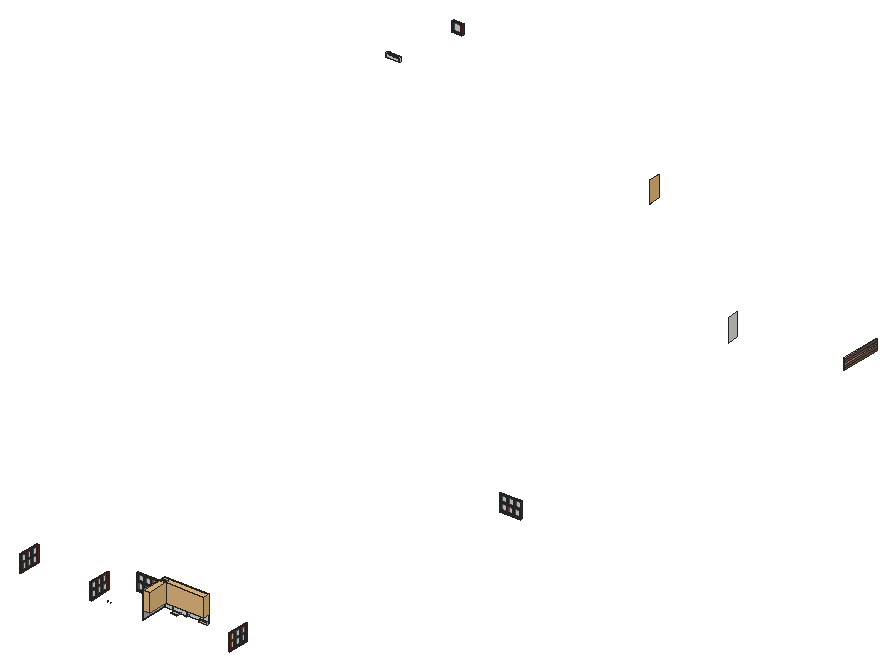
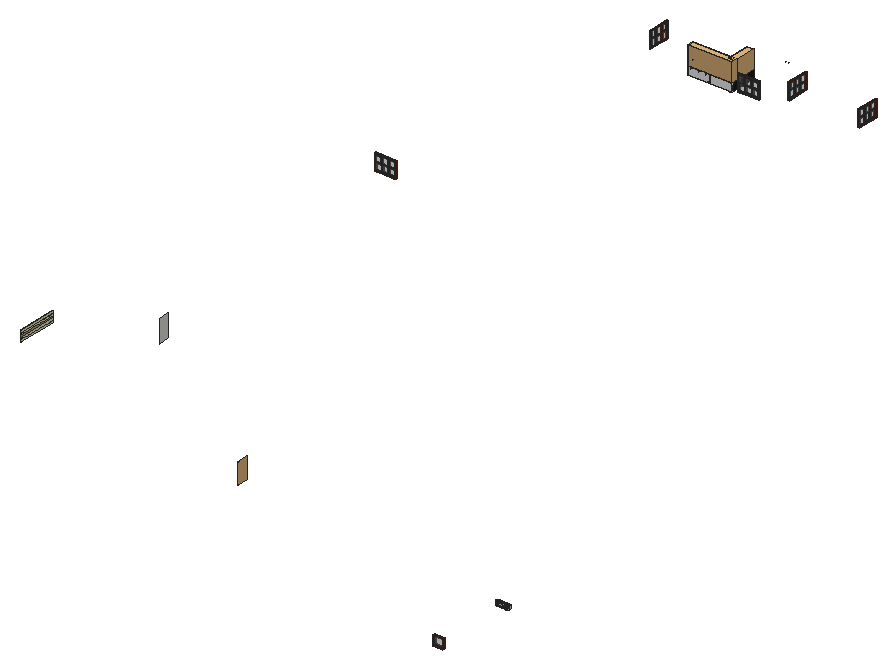
# SketchUp Ruby script. Lengths in inches.
U = 1.inch
M = Sketchup.active_model
def pt(a) = Geom::Point3d.new(a.map { |v| v * U })
def face(e, loops, mat)
  f = e.add_face(loops[0].map { |a| pt(a) })
  loops[1..].each { |l| e.add_face(l.map { |a| pt(a) }).erase! }
  f.material = f.back_material = mat if mat
  f
end
# faces: each face lists its corners as indices into pts; further lists are holes
def faces(e, pts, list, mat = nil) = list.each { |f| face(e, (f[0].is_a?(Array) ? f : [f]).map { |l| l.map { |i| pts[i] } }, mat) }
# xy, xz, yz: faces in a plane at the given z, y or x. An outline is a flat list of corners, or four numbers for a rectangle; further outlines are holes
def ring(l) = l.size == 4 ? [[l[0], l[1]], [l[2], l[1]], [l[2], l[3]], [l[0], l[3]]] : l.each_slice(2).to_a
def flat(e, list, mat, &to3) = list.each { |f| face(e, (f[0].is_a?(Array) ? f : [f]).map { |l| ring(l).map { |u, v| to3.(u, v) } }, mat) }
def xy(e, z, list, mat = nil) = flat(e, list, mat) { |x, y| [x, y, z] }
def xz(e, y, list, mat = nil) = flat(e, list, mat) { |x, z| [x, y, z] }
def yz(e, x, list, mat = nil) = flat(e, list, mat) { |y, z| [x, y, z] }
def lines(e, pts, list) = list.each { |a, b| e.add_line(pt(pts[a]), pt(pts[b])) }
# prism: a flat outline (further loops are holes) pulled along v
def prism(e, loops, v, mat = nil)
  f = face(e, loops, mat); d = Geom::Vector3d.new(v.map { |x| x * U })
  f.pushpull(f.normal.samedirection?(d) ? d.length : -d.length)
end
def box(e, o, s, mat = nil) = prism(e, [[o, [o[0] + s[0], o[1], o[2]], [o[0] + s[0], o[1] + s[1], o[2]], [o[0], o[1] + s[1], o[2]]]], [0, 0, s[2]], mat)
def at(x, y, z, deg = 0) = Geom::Transformation.translation(pt([x, y, z])) * Geom::Transformation.rotation(ORIGIN, Z_AXIS, deg.degrees)
def axes(o, x, y, z) = Geom::Transformation.new([*x, 0, *y, 0, *z, 0, *pt(o).to_a, 1])
def part(name) = M.definitions.add(name)
# library, detail: a bought-in or finely detailed component or shape, given as its bounding box
def library(name, o, s) = part(name).tap { |d| box(d.entities, o, s) }
def detail(e, o, s) = box(e.add_group.entities, o, s)
def put(e, d, t, mat = nil) = e.add_instance(d, t).tap { |i| i.material = mat if mat }
def group(e, t, mat = nil) = e.add_group.tap { |g| g.transformation = t; g.material = mat if mat }.entities
root = M.entities
M.materials.add("02 - Default1").color = [198, 154, 113]
M.materials.add("1").color = [234, 234, 196]
M.materials.add("3").color = [118, 89, 74]
M.materials.add("Material14 kitchen ceramic").color = [29, 29, 29]
M.materials.add("Material17 ceramic").color = [227, 223, 218]
M.materials.add("Material3 mirror").color = [229, 229, 229]
M.materials.add("Window Frame").color = [102, 40, 20]
M.materials.add("[Color_004]").color = [142, 142, 142]
M.materials.add("[Color_007]").color = [58, 58, 58]
M.materials.add("[Color_B17]").color = [102, 40, 20]
M.materials.add("[Color_C12]").color = [153, 91, 30]
M.materials.add("[Translucent Glass Gray]").color = [128, 128, 128]
M.materials["[Translucent Glass Gray]"].alpha = 0.44
M.materials.add("[Translucent_Glass_Gray]").color = [128, 128, 128]
M.materials["[Translucent_Glass_Gray]"].alpha = 0.5
M.materials.add("abu metal").color = [255, 255, 255]
M.materials.add("putih ceramic").color = [255, 255, 255]
c1 = library("Group\#63",[-80.46,-65.36,-92.6],[1.38,3.58,3.59])
c2 = part("Framed panel")
g1 = group(c2.entities,at(0,0,0))
prism(g1,[[[0,22.64,0],[21.26,22.64,0],[21.26,0,0],[0,0,0]],[[1.57,1.57,0],[19.69,1.57,0],[19.69,21.0625,0],[1.57,21.0625,0]]],[0,0,1.57],"[Color_B17]")
g2 = group(c2.entities,at(1.57,1.57,1.02))
xy(g2,0,[[0,0,18.11,19.49]],"[Translucent_Glass_Gray]")
c3 = part("Group\#25")
put(c3.entities,c2,at(0,21.0625,1.57))
put(c3.entities,c2,at(0,0,0))
c4 = part("Group\#47")
g3 = group(c4.entities,at(0,0,0))
prism(g3,[[[70.87,0,0],[0,0,0],[0,47.24,0],[70.87,47.24,0]],[[47.83,1.77,0],[69.09,1.77,0],[69.09,45.47,0],[47.83,45.47,0]],[[46.0625,45.47,0],[24.8,45.47,0],[24.8,1.77,0],[46.0625,1.77,0]],[[1.77,1.77,0],[23.03,1.77,0],[23.03,45.47,0],[1.77,45.47,0]]],[0,0,4.33],"[Color_B17]")
put(c4.entities,c3,at(1.77,1.77,0.59))
put(c4.entities,c3,at(24.8,1.77,0.59))
put(c4.entities,c3,at(47.83,1.77,0.59))
c5 = part("Component\#437")
prism(c5.entities,[[[0.59,0,2.2],[0.35,0,2.02],[0.16,0,1.77],[0.04,0,1.49],[0,0,1.18],[0.04,0,0.875],[0.16,0,0.59],[0.35,0,0.35],[0.59,0,0.16],[0.875,0,0.04],[1.18,0,0],[1.49,0,0.04],[1.77,0,0.16],[2.02,0,0.35],[2.2,0,0.59],[2.32,0,0.875],[2.36,0,1.18],[2.32,0,1.49],[2.2,0,1.77],[2.02,0,2.02],[1.77,0,2.2],[1.49,0,2.32],[1.18,0,2.36],[0.875,0,2.32]]],[0,0.47,0],"abu metal")
c6 = library("Kitchen cabinet run \#1",[0,0,-0.43],[99.61,27.56,87.04])
c7 = part("Component\#435")
box(c7.entities,[0,0,0],[113.78,0.2,35.43],"[Translucent Glass Gray]")
c8 = part("Component\#387")
xy(c8.entities,0,[[0,0,113.78,1.57]],"Material14 kitchen ceramic")
xy(c8.entities,35.43,[[0,0,113.78,1.57]],"Material14 kitchen ceramic")
xz(c8.entities,0,[[0,0,113.78,35.43]],"Material14 kitchen ceramic")
xz(c8.entities,1.57,[[0,0,113.78,35.43]],"Material17 ceramic")
yz(c8.entities,0,[[0,0,1.57,35.43]],"Material14 kitchen ceramic")
yz(c8.entities,113.78,[[0,0,1.57,35.43]],"Material14 kitchen ceramic")
c9 = library("Kitchen cabinet run",[0,0,-0.43],[27.56,188.98,87.04])
c10 = library("Gas cooktop",[0,0,0],[28.35,16.54,1.98])
c11 = part("Component\#432")
box(c11.entities,[-13.78,0,0],[13.78,19.88,0.79])
c12 = part("Component\#433")
box(c12.entities,[0,0,0],[13.78,35.71,0.79],"Material14 kitchen ceramic")
c13 = library("Sem+nome",[12.38,5.35,0],[34.47,6.17,9.61])
c14 = library("Deca_Torneira+Lavatorio+Clean_1178.C.CLN_Parede",[5.41,0,8.81],[3.41,8.24,3.84])
c15 = part("Component\#434")
xy(c15.entities,0,[[0,0,0.2,57.55]],"abu metal")
xy(c15.entities,35.43,[[0,0,0.2,57.55]],"abu metal")
xz(c15.entities,0,[[0,0,0.2,35.43]],"abu metal")
xz(c15.entities,57.55,[[0,0,0.2,35.43]],"abu metal")
yz(c15.entities,0,[[0,0,57.55,35.43]],"abu metal")
yz(c15.entities,0.2,[[0,0,57.55,35.43]],"Material3 mirror")
c16 = part("Component\#436")
prism(c16.entities,[[[0,1.96,0.29],[0,1.71,0.12],[0,1.41,0.02],[0,1.11,0],[0,0.8,0.06],[0,0.53,0.19],[0,0.29,0.4],[0,0.12,0.65],[0,0.02,0.94],[0,0,1.25],[0,0.06,1.55],[0,0.19,1.83],[0,0.4,2.0625],[0,0.65,2.24],[0,0.94,2.34],[0,1.25,2.36],[0,1.55,2.3],[0,1.83,2.16],[0,2.0625,1.96],[0,2.24,1.71],[0,2.34,1.41],[0,2.36,1.11],[0,2.3,0.8],[0,2.16,0.53]]],[0.12,0,0],"abu metal")
c17 = part("Component\#350")
xy(c17.entities,0,[[0,0,1.57,1.57],[0,1.57,1.57,188.98]],"putih ceramic")
xy(c17.entities,35.43,[[0,0,1.57,1.57],[0,1.57,1.57,188.98]],"putih ceramic")
xz(c17.entities,0,[[0,0,1.57,35.43]],"putih ceramic")
xz(c17.entities,1.57,[[0,0,1.57,35.43]],"putih ceramic")
xz(c17.entities,188.98,[[0,0,1.57,35.43]],"Material14 kitchen ceramic")
yz(c17.entities,0,[[0,0,1.57,35.43],[1.57,0,188.98,35.43]],"putih ceramic")
yz(c17.entities,1.57,[[0,0,1.57,35.43]],"Material14 kitchen ceramic")
yz(c17.entities,1.57,[[1.57,0,188.98,35.43]],"Material17 ceramic")
c18 = part("Group\#331")
xy(c18.entities,0,[[0,0,0.82,6.2]],"1")
xy(c18.entities,114.11,[[0,0,0.82,6.2]],"1")
xz(c18.entities,0,[[0,0,0.82,114.11]],"1")
xz(c18.entities,6.2,[[0,0,0.82,114.11]],"1")
yz(c18.entities,0,[[0,0,6.2,114.11]],"1")
yz(c18.entities,0.82,[[0,0,6.2,114.11]],"3")
c19 = part("Group\#330")
put(c19.entities,c18,axes([-0.82,0,0],[1,0,0],[0,1.45243,0],[0,0,1]),"1")
c20 = part("Group\#329")
box(c20.entities,[0,0,0],[0.82,6.2,114.11],"02 - Default1")
c21 = part("Group\#328")
put(c21.entities,c20,axes([-0.82,0,0],[1,0,0],[0,1.45243,0],[0,0,1]))
c22 = library("Group\#223",[0,0,0],[5,19.46,126.79])
c23 = library("Group\#73",[-80.34,-149.03,-93.91],[1.18,2.79,3])
c24 = library("Group\#74",[-80.34,-139.83,-93.89],[1.18,2.84,2.98])
g4 = group(root,at(1625.625,382,79.75))
prism(g4,[[[-15.5,7.07,-9.29],[-15.45,7.07,-9.6],[-15.52,7.07,-9.6],[-15.57,7.07,-9.29]]],[0,-0.1,0],"[Color_004]")
g5 = group(root,at(1625.625,382,79.75))
detail(g5,[-14.86,6.97,-9.37],[0.08,0.1,0.08])
put(root,c1,axes([1625.625,382.01,79.75],[0,-0.088,0],[0.10336,0,0],[0,0,0.10336]))
put(root,c4,axes([1540.13,478.85,36],[0,-0.87489,0],[0,0,1.016],[-1,0,0]))
put(root,c4,axes([1334.1,478.85,36],[0,-0.87489,0],[0,0,1.016],[-1,0,0]))
put(root,c5,axes([1678.38,448.75,42.65],[0,-0.69,0],[0.69,0,0],[0,0,0.69]))
put(root,c4,axes([1936.1875,427.84,36],[0,0.87489,0],[0,0,1.016],[1,0,0]))
put(root,c6,axes([1677.51,503.99,48.9],[0,-0.69,0],[0.69,0,0],[0,0,0.62727]))
put(root,c7,axes([1678.51,513.77,24.45],[0,-0.69,0],[0.69,0,0],[0,0,0.69]))
put(root,c8,axes([1677.51,513.77,24.45],[0,-0.69,0],[0.69,0,0],[0,0,0.69]))
put(root,c5,axes([1678.38,476.19,42.65],[0,-0.69,0],[0.69,0,0],[0,0,0.69]))
put(root,c5,axes([1678.38,504.28,42.65],[0,-0.69,0],[0.69,0,0],[0,0,0.69]))
put(root,c9,axes([1677.51,514.85,48.9],[0,-0.69,0],[0.69,0,0],[0,0,0.62727]))
put(root,c10,axes([1706.85,500.58,24.45],[0.69,0,0],[0,0.69,0],[0,0,0.69]))
put(root,c11,axes([1793.64,504.67,65.5],[0,-0.69,0],[0.69,0,0],[0,0,0.69]))
put(root,c12,axes([1768.06,514.17,68.67],[0,-0.69,0],[0.69,0,0],[0,0,0.69]))
put(root,c13,axes([1815.7,515.55,24.45],[-0.69,0,0],[0,-0.69,0],[0,0,0.69]))
put(root,c14,axes([1743.4,508.39,19.76],[0.6535,0,0],[0,0.6535,0],[0,0,0.6535]))
put(root,c15,axes([1703.45,513.77,24.45],[0,-0.69,0],[0.69,0,0],[0,0,0.69]))
put(root,c16,axes([1797.34,513.77,42.65],[0,-0.69,0],[0.69,0,0],[0,0,0.69]))
put(root,c16,axes([1690.41,513.77,42.65],[0,-0.69,0],[0.69,0,0],[0,0,0.69]))
put(root,c16,axes([1753.6,513.77,42.65],[0,-0.69,0],[0.69,0,0],[0,0,0.69]))
put(root,c16,axes([1775.58,513.77,42.65],[0,-0.69,0],[0.69,0,0],[0,0,0.69]))
put(root,c17,axes([1677.51,514.85,24.45],[0,-0.69,0],[0.69,0,0],[0,0,0.69]))
put(root,c4,axes([1654.61,518.23,36],[-0.87489,0,0],[0,0,1.016],[0,1,0]))
put(root,c4,axes([2076.07,1332.25,36],[-0.87489,0,0],[0,0,1.016],[0,1,0]))
g6 = group(root,at(1942.8125,2264.52,48.19))
yz(g6,0,[[0,0,32.75,65.92]])
put(root,c19,axes([2215.32,2470.24,31.98],[1,0,0],[0,0,0.67033],[0,-1.0271,0]),"02 - Default1")
put(root,c19,axes([2215.32,2470.24,38.15],[1,0,0],[0,0,0.67033],[0,-1.0271,0]),"02 - Default1")
put(root,c21,axes([2215.32,2470.24,44.6],[1,0,0],[0,0,0.67033],[0,-1.0271,0]),"02 - Default1")
put(root,c19,axes([2215.32,2470.24,50.83],[1,0,0],[0,0,0.67033],[0,-1.0271,0]),"02 - Default1")
put(root,c19,axes([2215.32,2470.24,57.25],[1,0,0],[0,0,0.67033],[0,-1.0271,0]),"02 - Default1")
put(root,c22,axes([1389.45,2666.85,44.99],[0.12,0,0],[0,1.68174,0],[0,0,0.4902]))
g7 = group(root,at(527.48,2794.13,79.75))
xy(g7,-12.74,[[-18.76,0,18.76,1.73]])
xy(g7,-2.26,[[-15.67,0.14,-11.93,0.35],[-11.73,0.14,-7.99,0.35],[-7.79,0.14,-4.04,0.35],[-3.84,0.14,-0.1,0.35],[0.1,0.14,3.84,0.35],
  [4.04,0.14,7.79,0.35],[7.99,0.14,11.73,0.35],[11.93,0.14,15.67,0.35],[-15.67,0.43,-11.93,0.64],[-11.73,0.43,-7.99,0.64],
  [-7.79,0.43,-4.04,0.64],[-3.84,0.43,-0.1,0.64],[0.1,0.43,3.84,0.64],[4.04,0.43,7.79,0.64],[7.99,0.43,11.73,0.64],
  [11.93,0.43,15.67,0.64],[-15.67,0.73,-11.93,0.93],[-11.73,0.73,-7.99,0.93],[-7.79,0.73,-4.04,0.93],[-3.84,0.73,-0.1,0.93],
  [0.1,0.73,3.84,0.93],[4.04,0.73,7.79,0.93],[7.99,0.73,11.73,0.93],[11.93,0.73,15.67,0.93]])
xy(g7,0,[[[-18.76,0,18.76,1.73],[4.04,0.73,4.04,0.93,11.73,0.93,11.73,0.73,7.99,0.73,7.99,0.93,7.79,0.93,7.79,0.73],[4.04,0.14,4.04,0.35,7.79,0.35,7.79,0.14,7.99,0.14,7.99,0.35,11.73,0.35,11.73,0.14],[11.93,0.43,15.67,0.64],[11.93,0.14,15.67,0.35],[11.93,0.73,15.67,0.93],[-15.67,0.73,-11.93,0.93],[-15.67,0.14,-11.93,0.35],[-15.67,0.43,-11.93,0.64],[4.04,0.43,7.79,0.64],[-7.79,0.14,-4.04,0.35],[-7.79,0.43,-4.04,0.64],[-7.79,0.73,-4.04,0.93],[7.99,0.43,11.73,0.64],[0.1,0.43,3.84,0.64],[0.1,0.14,3.84,0.35],[0.1,0.73,3.84,0.93],[-11.73,0.14,-7.99,0.35],[-11.73,0.73,-7.99,0.93],[-3.84,0.73,-0.1,0.93],[-3.84,0.43,-0.1,0.64],[-3.84,0.14,-0.1,0.35],[-11.73,0.43,-7.99,0.64]]])
xz(g7,0,[[-18.76,-12.74,18.76,0]])
xz(g7,0.14,[[-15.67,-2.26,-11.93,0],[-11.73,-2.26,-7.99,0],[-7.79,-2.26,-4.04,0],[-3.84,-2.26,-0.1,0],[0.1,-2.26,3.84,0],
  [4.04,-2.26,7.79,0],[7.99,-2.26,11.73,0],[11.93,-2.26,15.67,0]])
xz(g7,0.35,[[-15.67,-2.26,-11.93,0],[-11.73,-2.26,-7.99,0],[-7.79,-2.26,-4.04,0],[-3.84,-2.26,-0.1,0],[0.1,-2.26,3.84,0],
  [4.04,-2.26,7.79,0],[7.99,-2.26,11.73,0],[11.93,-2.26,15.67,0]])
xz(g7,0.43,[[-15.67,-2.26,-11.93,0],[-11.73,-2.26,-7.99,0],[-7.79,-2.26,-4.04,0],[-3.84,-2.26,-0.1,0],[0.1,-2.26,3.84,0],
  [4.04,-2.26,7.79,0],[7.99,-2.26,11.73,0],[11.93,-2.26,15.67,0]])
xz(g7,0.64,[[-15.67,-2.26,-11.93,0],[-11.73,-2.26,-7.99,0],[-7.79,-2.26,-4.04,0],[-3.84,-2.26,-0.1,0],[0.1,-2.26,3.84,0],
  [4.04,-2.26,7.79,0],[7.99,-2.26,11.73,0],[11.93,-2.26,15.67,0]])
xz(g7,0.73,[[-15.67,-2.26,-11.93,0],[-11.73,-2.26,-7.99,0],[-7.79,-2.26,-4.04,0],[-3.84,-2.26,-0.1,0],[0.1,-2.26,3.84,0],
  [4.04,-2.26,7.79,0],[7.99,-2.26,11.73,0],[11.93,-2.26,15.67,0]])
xz(g7,0.93,[[-15.67,-2.26,-11.93,0],[-11.73,-2.26,-7.99,0],[-7.79,-2.26,-4.04,0],[-3.84,-2.26,-0.1,0],[0.1,-2.26,3.84,0],
  [4.04,-2.26,7.79,0],[7.99,-2.26,11.73,0],[11.93,-2.26,15.67,0]])
xz(g7,1.73,[[-18.76,-12.74,18.76,0]])
yz(g7,-18.76,[[0,-12.74,1.73,0]])
yz(g7,-15.67,[[0.14,-2.26,0.35,0],[0.43,-2.26,0.64,0],[0.73,-2.26,0.93,0]])
yz(g7,-11.93,[[0.14,-2.26,0.35,0],[0.43,-2.26,0.64,0],[0.73,-2.26,0.93,0]])
yz(g7,-11.73,[[0.14,-2.26,0.35,0],[0.43,-2.26,0.64,0],[0.73,-2.26,0.93,0]])
yz(g7,-7.99,[[0.14,-2.26,0.35,0],[0.43,-2.26,0.64,0],[0.73,-2.26,0.93,0]])
yz(g7,-7.79,[[0.14,-2.26,0.35,0],[0.43,-2.26,0.64,0],[0.73,-2.26,0.93,0]])
yz(g7,-4.04,[[0.14,-2.26,0.35,0],[0.43,-2.26,0.64,0],[0.73,-2.26,0.93,0]])
yz(g7,-3.84,[[0.14,-2.26,0.35,0],[0.43,-2.26,0.64,0],[0.73,-2.26,0.93,0]])
yz(g7,-0.1,[[0.14,-2.26,0.35,0],[0.43,-2.26,0.64,0],[0.73,-2.26,0.93,0]])
yz(g7,0.1,[[0.14,-2.26,0.35,0],[0.43,-2.26,0.64,0],[0.73,-2.26,0.93,0]])
yz(g7,3.84,[[0.14,-2.26,0.35,0],[0.43,-2.26,0.64,0],[0.73,-2.26,0.93,0]])
yz(g7,4.04,[[0.14,-2.26,0.35,0],[0.43,-2.26,0.64,0],[0.73,-2.26,0.93,0]])
yz(g7,7.79,[[0.14,-2.26,0.35,0],[0.43,-2.26,0.64,0],[0.73,-2.26,0.93,0]])
yz(g7,7.99,[[0.14,-2.26,0.35,0],[0.43,-2.26,0.64,0],[0.73,-2.26,0.93,0]])
yz(g7,11.73,[[0.14,-2.26,0.35,0],[0.43,-2.26,0.64,0],[0.73,-2.26,0.93,0]])
yz(g7,11.93,[[0.14,-2.26,0.35,0],[0.43,-2.26,0.64,0],[0.73,-2.26,0.93,0]])
yz(g7,15.67,[[0.14,-2.26,0.35,0],[0.43,-2.26,0.64,0],[0.73,-2.26,0.93,0]])
yz(g7,18.76,[[0,-12.74,1.73,0]])
g8 = group(root,at(527.48,2794.13,79.75))
xy(g8,-12.74,[[-18.76,1.73,-15.875,5.65],[15.875,1.73,18.76,5.65]])
xy(g8,-9.91,[[-15.875,1.73,15.875,7.03]])
xy(g8,-9.7,[[-3.48,6.93,3.48,7.03]])
xy(g8,-9.07,[[-3.48,6.93,3.48,7.03]])
xy(g8,-8.96,[[-15.875,7.03,15.875,7.62],[-18.76,7.62,-15.875,7.73],[15.875,7.62,18.76,7.73]])
xy(g8,0,[[-18.76,1.73,18.76,5.65]])
xz(g8,1.73,[[-18.76,-12.74,-15.875,-12.74,-15.875,-9.91,15.875,-9.91,15.875,-12.74,18.76,-12.74,18.76,0,-18.76,0]])
xz(g8,5.65,[[-18.76,-0.12,18.76,0]])
xz(g8,6.93,[[-3.48,-9.7,3.48,-9.07]],"[Color_007]")
xz(g8,7.03,[[[-15.875,-9.91,15.875,-8.96],[-3.48,-9.7,3.48,-9.07]]])
xz(g8,7.62,[[-18.76,-8.96,18.76,-2.44]])
xz(g8,7.73,[[-18.76,-10.29,-15.875,-8.96],[15.875,-10.29,18.76,-8.96]])
yz(g8,-18.76,[[1.73,-12.74,1.73,0,5.65,0,5.65,-0.12,5.96,-0.15,6.26,-0.24,6.54,-0.375,6.81,-0.57,7.04,-0.8,7.24,-1.08,7.41,-1.39,7.53,-1.72,7.6,-2.08,7.62,-2.44,7.62,-8.96,7.73,-8.96,7.73,-10.29,7.7,-10.68,7.625,-11.05,7.5,-11.4,7.33,-11.73,7.12,-12.02,6.87,-12.27,6.59,-12.47,6.29,-12.62,5.97,-12.71,5.65,-12.74]])
yz(g8,-15.875,[[1.73,-12.74,5.65,-12.74,5.97,-12.71,6.29,-12.62,6.59,-12.47,6.87,-12.27,7.12,-12.02,7.33,-11.73,7.5,-11.4,7.625,-11.05,7.7,-10.68,7.73,-10.29,7.73,-8.96,7.03,-8.96,7.03,-9.91,1.73,-9.91]])
yz(g8,-3.48,[[6.93,-9.7,7.03,-9.07]])
yz(g8,3.48,[[6.93,-9.7,7.03,-9.07]])
yz(g8,15.875,[[1.73,-12.74,1.73,-9.91,7.03,-9.91,7.03,-8.96,7.73,-8.96,7.73,-10.29,7.7,-10.68,7.625,-11.05,7.5,-11.4,7.33,-11.73,7.12,-12.02,6.87,-12.27,6.59,-12.47,6.29,-12.62,5.97,-12.71,5.65,-12.74]])
yz(g8,18.76,[[1.73,-12.74,5.65,-12.74,5.97,-12.71,6.29,-12.62,6.59,-12.47,6.87,-12.27,7.12,-12.02,7.33,-11.73,7.5,-11.4,7.625,-11.05,7.7,-10.68,7.73,-10.29,7.73,-8.96,7.62,-8.96,7.62,-2.44,7.6,-2.08,7.53,-1.72,7.41,-1.39,7.24,-1.08,7.04,-0.8,6.81,-0.57,6.54,-0.375,6.26,-0.24,5.96,-0.15,5.65,-0.12,5.65,0,1.73,0]])
p = [[-15.875,5.65,-12.74],[-18.76,5.65,-12.74],[-18.76,5.97,-12.71],[-15.875,5.97,-12.71],[18.76,5.65,-12.74],[15.875,5.65,-12.74],
  [15.875,5.97,-12.71],[18.76,5.97,-12.71],[-18.76,6.29,-12.62],[-15.875,6.29,-12.62],[15.875,6.29,-12.62],[18.76,6.29,-12.62],
  [-15.875,6.59,-12.47],[-18.76,6.59,-12.47],[15.875,6.59,-12.47],[18.76,6.59,-12.47],[-18.76,6.87,-12.27],[-15.875,6.87,-12.27],
  [15.875,6.87,-12.27],[18.76,6.87,-12.27],[-18.76,7.12,-12.02],[-15.875,7.12,-12.02],[15.875,7.12,-12.02],[18.76,7.12,-12.02],
  [-18.76,7.33,-11.73],[-15.875,7.33,-11.73],[15.875,7.33,-11.73],[18.76,7.33,-11.73],[-18.76,7.5,-11.4],[-15.875,7.5,-11.4],
  [15.875,7.5,-11.4],[18.76,7.5,-11.4],[-15.875,7.625,-11.05],[-18.76,7.625,-11.05],[15.875,7.625,-11.05],[18.76,7.625,-11.05],
  [-18.76,7.7,-10.68],[-15.875,7.7,-10.68],[15.875,7.7,-10.68],[18.76,7.7,-10.68],[-18.76,7.73,-10.29],[-15.875,7.73,-10.29],
  [15.875,7.73,-10.29],[18.76,7.73,-10.29],[18.76,7.62,-2.44],[-18.76,7.62,-2.44],[-18.76,7.6,-2.08],[18.76,7.6,-2.08],
  [-18.76,7.53,-1.72],[18.76,7.53,-1.72],[18.76,7.41,-1.39],[-18.76,7.41,-1.39],[-18.76,7.24,-1.08],[18.76,7.24,-1.08],
  [-18.76,7.04,-0.8],[18.76,7.04,-0.8],[-18.76,6.81,-0.57],[18.76,6.81,-0.57],[-18.76,6.54,-0.375],[18.76,6.54,-0.375],
  [18.76,6.26,-0.24],[-18.76,6.26,-0.24],[-18.76,5.65,-0.12],[18.76,5.65,-0.12],[18.76,5.96,-0.15],[-18.76,5.96,-0.15]]
faces(g8,p,[[0,1,2,3],[4,5,6,7],[8,9,3,2],[10,11,7,6],[12,9,8,13],[10,14,15,11],[12,13,16,17],[15,14,18,19],
  [20,21,17,16],[22,23,19,18],[21,20,24,25],[23,22,26,27],[28,29,25,24],[30,31,27,26],[32,29,28,33],[30,34,35,31],
  [32,33,36,37],[35,34,38,39],[40,41,37,36],[42,43,39,38],[44,45,46,47],[48,49,47,46],[50,49,48,51],[50,51,52,53],
  [54,55,53,52],[55,54,56,57],[58,59,57,56],[60,59,58,61],[62,63,64,65],[60,61,65,64]])
g9 = group(root,at(527.48,2794.13,79.75))
xy(g9,-12.375,[[-15.875,3.67,15.875,5.58]])
xy(g9,-10.42,[[-15.875,7,-9.1,7.25],[-8.85,7,4.71,7.25],[4.95,7,15.875,7.25]])
xy(g9,-9.91,[[-15.875,3.67,15.875,3.67,15.875,7,4.95,7,4.95,7.25,4.71,7.25,4.71,7,-8.85,7,-8.85,7.25,-9.1,7.25,-9.1,7,-15.875,7]])
xz(g9,3.67,[[-15.875,-12.375,15.875,-9.91]])
xz(g9,7,[[-15.875,-10.42,-9.1,-9.91],[-8.85,-10.42,4.71,-9.91],[4.95,-10.42,15.875,-9.91]],"[Color_007]")
xz(g9,7.25,[[-9.1,-10.42,-8.85,-9.91],[4.71,-10.42,4.95,-9.91]])
yz(g9,-15.875,[[3.67,-12.375,3.67,-9.91,7,-9.91,7,-10.42,7.25,-10.42,7.24,-10.46,7.23,-10.73,7.17,-11.02,7.07,-11.31,6.93,-11.57,6.76,-11.8,6.5625,-12,6.34,-12.16,6.1,-12.28,5.84,-12.35,5.58,-12.375]])
yz(g9,-9.1,[[7,-10.42,7.25,-9.91]])
yz(g9,-8.85,[[7,-10.42,7.25,-9.91]])
yz(g9,4.71,[[7,-10.42,7.25,-9.91]])
yz(g9,4.95,[[7,-10.42,7.25,-9.91]])
yz(g9,15.875,[[3.67,-12.375,5.58,-12.375,5.84,-12.35,6.1,-12.28,6.34,-12.16,6.5625,-12,6.76,-11.8,6.93,-11.57,7.07,-11.31,7.17,-11.02,7.23,-10.73,7.24,-10.46,7.25,-10.42,7,-10.42,7,-9.91,3.67,-9.91]])
p = [[15.875,5.58,-12.375],[-15.875,5.58,-12.375],[-15.875,5.84,-12.35],[15.875,5.84,-12.35],[-15.875,6.1,-12.28],[15.875,6.1,-12.28],
  [15.875,6.34,-12.16],[-15.875,6.34,-12.16],[-15.875,6.5625,-12],[15.875,6.5625,-12],[-15.875,6.76,-11.8],[15.875,6.76,-11.8],
  [-15.875,6.93,-11.57],[15.875,6.93,-11.57],[-15.875,7.07,-11.31],[15.875,7.07,-11.31],[15.875,7.17,-11.02],[-15.875,7.17,-11.02],
  [-15.875,7.23,-10.73],[15.875,7.23,-10.73],[-15.875,7.24,-10.46],[-9.1,7.24,-10.46],[-8.85,7.24,-10.46],[4.71,7.24,-10.46],
  [4.95,7.24,-10.46],[15.875,7.24,-10.46],[15.875,7.25,-10.42],[-15.875,7.25,-10.42],[-9.1,7.25,-10.42],[-8.85,7.25,-10.42],
  [4.71,7.25,-10.42],[4.95,7.25,-10.42]]
faces(g9,p,[[0,1,2,3],[4,5,3,2],[6,5,4,7],[6,7,8,9],[10,11,9,8],[11,10,12,13],[14,15,13,12],[16,15,14,17],
  [16,17,18,19],[18,20,21,22,23,24,25,19]])
faces(g9,p,[[26,25,24,23,22,21,20,27,28,29,30,31]],"[Color_C12]")
g10 = group(root,at(527.48,2794.13,79.75))
prism(g10,[[[18.74,7.73,-8.96],[18.74,7.73,-2.44],[18.74,7.7,-2.06],[18.74,7.625,-1.6875],[18.74,7.5,-1.33],[18.74,7.33,-1.01],[18.74,7.12,-0.72],[18.74,6.87,-0.47],[18.74,6.59,-0.27],[18.74,6.29,-0.12],[18.74,5.97,-0.03],[18.74,5.65,0],[18.74,5.65,-0.12],[18.74,5.96,-0.15],[18.74,6.26,-0.24],[18.74,6.54,-0.375],[18.74,6.81,-0.57],[18.74,7.04,-0.8],[18.74,7.24,-1.08],[18.74,7.41,-1.39],[18.74,7.53,-1.72],[18.74,7.6,-2.08],[18.74,7.62,-2.44],[18.74,7.62,-8.96]]],[-37.47,0,0])
put(root,c23,axes([527.48,2794.19,79.75],[0,-0.088,0],[0.10336,0,0],[0,0,0.10336]))
g11 = group(root,at(527.48,2794.19,79.75))
detail(g11,[-15.51,6.97,-9.71],[0.08,0.1,0.08])
g12 = group(root,at(527.48,2794.19,79.75))
detail(g12,[-14.73,6.97,-9.7],[0.25,0.1,0.41])
put(root,c24,axes([527.48,2794.19,79.75],[0,-0.088,0],[0.10336,0,0],[0,0,0.10336]))
g13 = group(root,at(527.48,2794.19,79.75),"[Color_004]")
prism(g13,[[[-15.07,7.07,-9.4],[-14.96,7.07,-9.6],[-14.92,7.07,-9.4],[-14.85,7.07,-9.4],[-14.91,7.07,-9.7],[-14.98,7.07,-9.7],[-15.15,7.07,-9.4]]],[0,-0.1,0],"[Color_004]")
g14 = group(root,at(527.48,2794.19,79.75))
prism(g14,[[[-14.79,7.07,-9.7],[-14.84,7.07,-9.4],[-14.77,7.07,-9.4],[-14.72,7.07,-9.7]]],[0,-0.1,0],"[Color_004]")
g15 = group(root,at(527.48,2794.19,79.75))
prism(g15,[[[-15.5,7.07,-9.29],[-15.45,7.07,-9.6],[-15.52,7.07,-9.6],[-15.57,7.07,-9.29]]],[0,-0.1,0],"[Color_004]")
g16 = group(root,at(527.48,2794.19,79.75))
detail(g16,[-14.86,6.97,-9.37],[0.08,0.1,0.08])
put(root,c1,axes([527.48,2794.21,79.75],[0,-0.088,0],[0.10336,0,0],[0,0,0.10336]))
g17 = group(root,at(561.25,3013.2,48.1875))
g18 = group(g17,at(0,0,0))
prism(g18,[[[0,0,29.53],[0,0,0],[-29.53,0,0],[-29.53,0,29.53]],[[-1.77,0,1.77],[-1.77,0,27.76],[-27.76,0,27.76],[-27.76,0,1.77]]],[0,-4.33,0],"Window Frame")
g19 = group(g17,at(-1.77,-1.97,1.77))
g20 = group(g19,at(0,0,0))
prism(g20,[[[0,0,25.98],[0,0,0],[-25.98,0,0],[-25.98,0,25.98]],[[-24.41,0,1.57],[-1.57,0,1.57],[-1.57,0,24.41],[-24.41,0,24.41]]],[0,-1.57,0],"Window Frame")
g21 = group(g19,at(-1.57,-0.91,1.57))
xz(g21,0,[[-22.83,0,0,22.83]],"[Translucent_Glass_Gray]")
